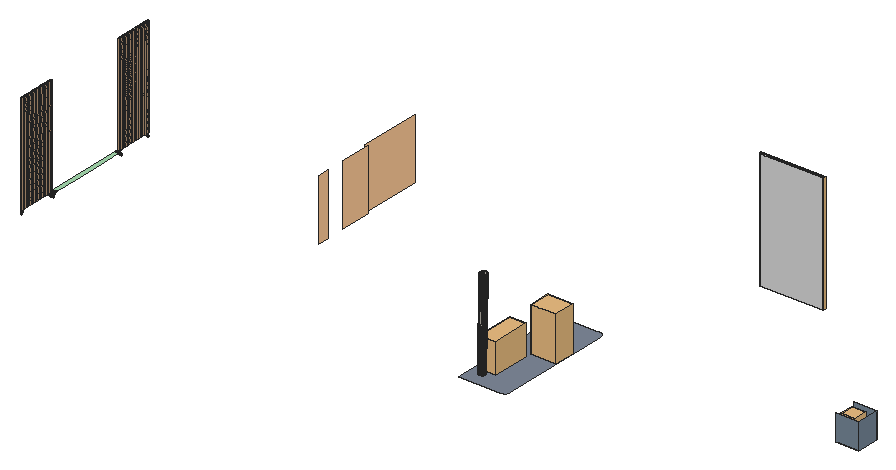
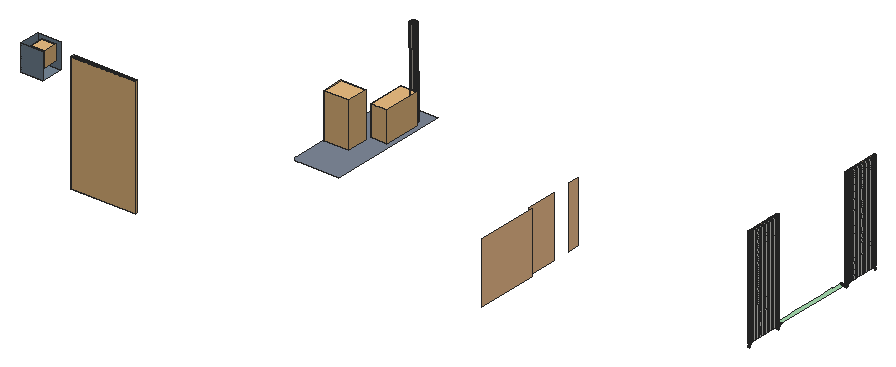
# SketchUp Ruby script. Lengths in inches.
U = 1.inch
M = Sketchup.active_model
def pt(a) = Geom::Point3d.new(a.map { |v| v * U })
def face(e, loops, mat)
  f = e.add_face(loops[0].map { |a| pt(a) })
  loops[1..].each { |l| e.add_face(l.map { |a| pt(a) }).erase! }
  f.material = f.back_material = mat if mat
  f
end
# faces: each face lists its corners as indices into pts; further lists are holes
def faces(e, pts, list, mat = nil) = list.each { |f| face(e, (f[0].is_a?(Array) ? f : [f]).map { |l| l.map { |i| pts[i] } }, mat) }
# xy, xz, yz: faces in a plane at the given z, y or x. An outline is a flat list of corners, or four numbers for a rectangle; further outlines are holes
def ring(l) = l.size == 4 ? [[l[0], l[1]], [l[2], l[1]], [l[2], l[3]], [l[0], l[3]]] : l.each_slice(2).to_a
def flat(e, list, mat, &to3) = list.each { |f| face(e, (f[0].is_a?(Array) ? f : [f]).map { |l| ring(l).map { |u, v| to3.(u, v) } }, mat) }
def xy(e, z, list, mat = nil) = flat(e, list, mat) { |x, y| [x, y, z] }
def xz(e, y, list, mat = nil) = flat(e, list, mat) { |x, z| [x, y, z] }
def yz(e, x, list, mat = nil) = flat(e, list, mat) { |y, z| [x, y, z] }
def lines(e, pts, list) = list.each { |a, b| e.add_line(pt(pts[a]), pt(pts[b])) }
# prism: a flat outline (further loops are holes) pulled along v
def prism(e, loops, v, mat = nil)
  f = face(e, loops, mat); d = Geom::Vector3d.new(v.map { |x| x * U })
  f.pushpull(f.normal.samedirection?(d) ? d.length : -d.length)
end
def box(e, o, s, mat = nil) = prism(e, [[o, [o[0] + s[0], o[1], o[2]], [o[0] + s[0], o[1] + s[1], o[2]], [o[0], o[1] + s[1], o[2]]]], [0, 0, s[2]], mat)
def at(x, y, z, deg = 0) = Geom::Transformation.translation(pt([x, y, z])) * Geom::Transformation.rotation(ORIGIN, Z_AXIS, deg.degrees)
def axes(o, x, y, z) = Geom::Transformation.new([*x, 0, *y, 0, *z, 0, *pt(o).to_a, 1])
def part(name) = M.definitions.add(name)
# library, detail: a bought-in or finely detailed component or shape, given as its bounding box
def library(name, o, s) = part(name).tap { |d| box(d.entities, o, s) }
def detail(e, o, s) = box(e.add_group.entities, o, s)
def put(e, d, t, mat = nil) = e.add_instance(d, t).tap { |i| i.material = mat if mat }
def group(e, t, mat = nil) = e.add_group.tap { |g| g.transformation = t; g.material = mat if mat }.entities
root = M.entities
M.materials.add("Leather K01 Brown 12cm").color = [167, 219, 175]
M.materials.add("Plywood B 50cm").color = [193, 159, 125]
M.materials.add("Stone E 150cm").color = [186, 180, 170]
M.materials.add("[0110_LightSlateGray]").color = [127, 136, 153]
M.materials.add("[0110_LightSlateGray]1").color = [119, 136, 153]
M.materials.add("[Color A01]1").color = [216, 216, 216]
M.materials.add("[Color C02]").color = [255, 204, 153]
c1 = library("Group\#9",[-0.5,-0.5,0],[47.92,1.3125,88])
c2 = library("Books 120 040",[-9.2,-4.08,-0.03],[18.37,8.13,11.52])
c3 = library("Vase 160 010",[-6.09,-4.45,0],[12.18,8.9,22.13])
c4 = library("Spot Light\#1",[-5.1,-5.1,-11.05],[10.2,10.2,11.05])
xy(root,57.82,[[536.14,116.57,553.2,132.48]],"[0110_LightSlateGray]1")
xy(root,62.4375,[[391.15,226.6,438.07,227.79]],"[Color A01]1")
xy(root,63.71,[[[323.37,31.6,353.74,31.6,354.39,31.64,355.03,31.75,355.65,31.9375,356.24,32.19,356.78,32.51,357.28,32.89,357.71,33.33,358.07,33.8,358.36,34.32,358.57,34.86,358.7,35.43,358.74,36,358.74,119.11,358.7,119.68,358.57,120.25,358.36,120.79,358.07,121.31,357.71,121.79,357.28,122.22,356.78,122.6,356.24,122.92,355.65,123.17,355.03,123.36,354.39,123.47,353.74,123.51,323.37,123.51],[331.76,40.57,331.08,40.64,330.44,40.87,329.89,41.24,329.47,41.71,329.21,42.27,329.12,42.87,329.2,43.46,329.46,44.02,329.875,44.5,330.41,44.87,331.05,45.11,331.72,45.1875,332.4,45.11,333.04,44.89,333.59,44.52,334.01,44.05,334.27,43.49,334.37,42.89,334.28,42.29,334.02,41.74,333.61,41.25,333.07,40.89,332.43,40.65]]],"[0110_LightSlateGray]")
xy(root,70.0625,[[8.12,18.51,9.37,19.28],[8.12,21.51,9.37,21.77],[9.37,21.51,9.43,21.51,9.43,42.51,9.37,42.51,9.37,42.15,8.12,42.15,8.12,41.68,9.37,41.68,9.37,40.91,8.12,40.91,8.12,40.43,9.37,40.43,9.37,39.66,8.12,39.66,8.12,39.1875,9.37,39.1875,9.37,38.42,8.12,38.42,8.12,37.94,9.37,37.94,9.37,37.18,8.12,37.18,8.12,36.7,9.37,36.7,9.37,35.93,8.12,35.93,8.12,35.45,9.37,35.45,9.37,34.6875,8.12,34.6875,8.12,34.21,9.37,34.21,9.37,33.44,8.12,33.44,8.12,32.97,9.37,32.97,9.37,32.2,8.12,32.2,8.12,31.72,9.37,31.72,9.37,30.95,8.12,30.95,8.12,30.48,9.37,30.48,9.37,29.71,8.12,29.71,8.12,29.23,9.37,29.23,9.37,28.47,8.12,28.47,8.12,27.99,9.37,27.99,9.37,27.22,8.12,27.22,8.12,26.74,9.37,26.74,9.37,25.98,8.12,25.98,8.12,25.5,9.37,25.5,9.37,24.73,8.12,24.73,8.12,24.25,9.37,24.25,9.37,23.49,8.12,23.49,8.12,23.01,9.37,23.01,9.37,22.24,8.12,22.24,8.12,21.77,9.37,21.77],[8.12,22.24,9.37,23.01],[8.12,23.49,9.37,24.25],
  [8.12,24.73,9.37,25.5],[8.12,25.98,9.37,26.74],[8.12,27.22,9.37,27.99],[8.12,28.47,9.37,29.23],[8.12,29.71,9.37,30.48],
  [8.12,30.95,9.37,31.72],[8.12,32.2,9.37,32.97],[8.12,33.44,9.37,34.21],[8.12,34.6875,9.37,35.45],[8.12,35.93,9.37,36.7],
  [8.12,37.18,9.37,37.94],[8.12,38.42,9.37,39.1875],[8.12,39.66,9.37,40.43],[8.12,40.91,9.37,41.68],[8.12,42.15,9.37,42.51],
  [8.12,112.01,9.37,112.23],[8.12,112.69,9.37,113.46],[8.12,113.92,9.37,114.6875],[8.12,115.15,9.37,115.91],[8.12,116.375,9.37,117.14],
  [8.12,117.6,9.37,118.37],[8.12,118.83,9.37,119.6],[8.12,120.06,9.37,120.82],[8.12,121.28,9.37,122.05],[8.12,122.51,9.37,123.28],
  [8.12,123.74,9.37,124.5],[8.12,124.97,9.37,125.73],[8.12,126.19,9.37,126.96],[8.12,127.42,9.37,128.1875],[8.12,128.65,9.37,129.41],
  [8.12,129.875,9.37,130.64],[8.12,131.1,9.37,131.87],[8.12,132.33,9.37,133.01]])
xy(root,70.0625,[[8.12,48.51,11.43,48.51,11.43,54.26,10.74,54.26,10.74,55.26,11.43,55.26,11.43,62.26,10.74,62.26,10.74,63.26,11.43,63.26,11.43,91.64,10.74,91.64,10.74,92.64,11.43,92.64,11.43,99.64,10.74,99.64,10.74,100.64,11.43,100.64,11.43,106.01,8.12,106.01],[9.37,112.01,9.43,112.01,9.43,133.01,9.37,133.01,9.37,132.33,8.12,132.33,8.12,131.87,9.37,131.87,9.37,131.1,8.12,131.1,8.12,130.64,9.37,130.64,9.37,129.875,8.12,129.875,8.12,129.41,9.37,129.41,9.37,128.65,8.12,128.65,8.12,128.1875,9.37,128.1875,9.37,127.42,8.12,127.42,8.12,126.96,9.37,126.96,9.37,126.19,8.12,126.19,8.12,125.73,9.37,125.73,9.37,124.97,8.12,124.97,8.12,124.5,9.37,124.5,9.37,123.74,8.12,123.74,8.12,123.28,9.37,123.28,9.37,122.51,8.12,122.51,8.12,122.05,9.37,122.05,9.37,121.28,8.12,121.28,8.12,120.82,9.37,120.82,9.37,120.06,8.12,120.06,8.12,119.6,9.37,119.6,9.37,118.83,8.12,118.83,8.12,118.37,9.37,118.37,9.37,117.6,8.12,117.6,8.12,117.14,9.37,117.14,9.37,116.375,8.12,116.375,8.12,115.91,9.37,115.91,9.37,115.15,8.12,115.15,8.12,114.6875,9.37,114.6875,9.37,113.92,8.12,113.92,8.12,113.46,9.37,113.46,9.37,112.69,8.12,112.69,8.12,112.23,9.37,112.23]],"Leather K01 Brown 12cm")
xy(root,144.0625,[[8.12,19.76,9.37,20.52],[8.12,43.4,9.37,44.16],[8.12,44.64,9.37,45.41],[8.12,45.89,9.37,46.65],[8.12,109.01,9.37,109.78],
  [8.12,110.24,9.37,111],[8.12,133.56,9.37,134.32],[8.12,134.78,9.37,135.55],[8.12,136.01,9.37,136.78]],"Plywood B 50cm")
xy(root,150.4375,[[391.15,226.6,438.07,227.79]],"[Color A01]1")
xz(root,18.51,[[8.12,70.0625,9.37,144.0625]],"Plywood B 50cm")
xz(root,19.28,[[8.12,70.0625,9.37,144.0625]],"Plywood B 50cm")
xz(root,19.76,[[8.12,70.0625,9.37,144.0625]],"Plywood B 50cm")
xz(root,20.52,[[8.12,70.0625,9.37,144.0625]],"Plywood B 50cm")
xz(root,21,[[8.12,70.0625,9.37,144.0625]],"Plywood B 50cm")
xz(root,21.77,[[8.12,70.0625,9.37,144.0625]],"Plywood B 50cm")
xz(root,22.24,[[8.12,70.0625,9.37,144.0625]],"Plywood B 50cm")
xz(root,23.01,[[8.12,70.0625,9.37,144.0625]],"Plywood B 50cm")
xz(root,23.49,[[8.12,70.0625,9.37,144.0625]],"Plywood B 50cm")
xz(root,24.25,[[8.12,70.0625,9.37,144.0625]],"Plywood B 50cm")
xz(root,24.73,[[8.12,70.0625,9.37,144.0625]],"Plywood B 50cm")
xz(root,25.5,[[8.12,70.0625,9.37,144.0625]])
xz(root,25.98,[[8.12,70.0625,9.37,144.0625]],"Plywood B 50cm")
xz(root,26.74,[[8.12,70.0625,9.37,144.0625]],"Plywood B 50cm")
xz(root,27.22,[[8.12,70.0625,9.37,144.0625]],"Plywood B 50cm")
xz(root,27.99,[[8.12,70.0625,9.37,144.0625]],"Plywood B 50cm")
xz(root,28.47,[[8.12,70.0625,9.37,144.0625]],"Plywood B 50cm")
xz(root,29.23,[[8.12,70.0625,9.37,144.0625]],"Plywood B 50cm")
xz(root,29.71,[[8.12,70.0625,9.37,144.0625]],"Plywood B 50cm")
xz(root,30.48,[[8.12,70.0625,9.37,144.0625]],"Plywood B 50cm")
xz(root,30.95,[[8.12,70.0625,9.37,144.0625]],"Plywood B 50cm")
xz(root,31.72,[[8.12,70.0625,9.37,144.0625]],"Plywood B 50cm")
xz(root,32.2,[[8.12,70.0625,9.37,144.0625]],"Plywood B 50cm")
xz(root,32.97,[[8.12,70.0625,9.37,144.0625]],"Plywood B 50cm")
xz(root,33.44,[[8.12,70.0625,9.37,144.0625]],"Plywood B 50cm")
xz(root,34.21,[[8.12,70.0625,9.37,144.0625]],"Plywood B 50cm")
xz(root,34.6875,[[8.12,70.0625,9.37,144.0625]],"Plywood B 50cm")
xz(root,35.45,[[8.12,70.0625,9.37,144.0625]],"Plywood B 50cm")
xz(root,35.93,[[8.12,70.0625,9.37,144.0625]],"Plywood B 50cm")
xz(root,36.7,[[8.12,70.0625,9.37,144.0625]],"Plywood B 50cm")
xz(root,37.18,[[8.12,70.0625,9.37,144.0625]],"Plywood B 50cm")
xz(root,37.94,[[8.12,70.0625,9.37,144.0625]],"Plywood B 50cm")
xz(root,38.42,[[8.12,70.0625,9.37,144.0625]],"Plywood B 50cm")
xz(root,39.1875,[[8.12,70.0625,9.37,144.0625]],"Plywood B 50cm")
xz(root,39.66,[[8.12,70.0625,9.37,144.0625]],"Plywood B 50cm")
xz(root,40.43,[[8.12,70.0625,9.37,144.0625]],"Plywood B 50cm")
xz(root,40.91,[[8.12,70.0625,9.37,144.0625]],"Plywood B 50cm")
xz(root,41.68,[[8.12,70.0625,9.37,144.0625]],"Plywood B 50cm")
xz(root,42.15,[[8.12,70.0625,9.37,144.0625]],"Plywood B 50cm")
xz(root,42.92,[[8.12,70.0625,9.37,144.0625]],"Plywood B 50cm")
xz(root,43.4,[[8.12,70.0625,9.37,144.0625]],"Plywood B 50cm")
xz(root,44.16,[[8.12,70.0625,9.37,144.0625]],"Plywood B 50cm")
xz(root,44.64,[[8.12,70.0625,9.37,144.0625]],"Plywood B 50cm")
xz(root,45.41,[[8.12,70.0625,9.37,144.0625]],"Plywood B 50cm")
xz(root,45.89,[[8.12,70.0625,9.37,144.0625]],"Plywood B 50cm")
xz(root,46.65,[[8.12,70.0625,9.37,144.0625]],"Plywood B 50cm")
xz(root,109.01,[[8.12,70.0625,9.37,144.0625]],"Plywood B 50cm")
xz(root,109.78,[[8.12,70.0625,9.37,144.0625]],"Plywood B 50cm")
xz(root,110.24,[[8.12,70.0625,9.37,144.0625]],"Plywood B 50cm")
xz(root,111,[[8.12,70.0625,9.37,144.0625]],"Plywood B 50cm")
xz(root,111.47,[[8.12,70.0625,9.37,144.0625]],"Plywood B 50cm")
xz(root,112.23,[[8.12,70.0625,9.37,144.0625]],"Plywood B 50cm")
xz(root,112.69,[[8.12,70.0625,9.37,144.0625]],"Plywood B 50cm")
xz(root,113.46,[[8.12,70.0625,9.37,144.0625]],"Plywood B 50cm")
xz(root,113.92,[[8.12,70.0625,9.37,144.0625]],"Plywood B 50cm")
xz(root,114.6875,[[8.12,70.0625,9.37,144.0625]],"Plywood B 50cm")
xz(root,115.15,[[8.12,70.0625,9.37,144.0625]],"Plywood B 50cm")
xz(root,115.91,[[8.12,70.0625,9.37,144.0625]],"Plywood B 50cm")
xz(root,116.375,[[8.12,70.0625,9.37,144.0625]],"Plywood B 50cm")
xz(root,116.57,[[536.14,57.82,553.2,76.9375]],"[0110_LightSlateGray]1")
xz(root,117.14,[[8.12,70.0625,9.37,144.0625]],"Plywood B 50cm")
xz(root,117.6,[[8.12,70.0625,9.37,144.0625]],"Plywood B 50cm")
xz(root,118.37,[[8.12,70.0625,9.37,144.0625]],"Plywood B 50cm")
xz(root,118.83,[[8.12,70.0625,9.37,144.0625]],"Plywood B 50cm")
xz(root,119.6,[[8.12,70.0625,9.37,144.0625]],"Plywood B 50cm")
xz(root,120.06,[[8.12,70.0625,9.37,144.0625]],"Plywood B 50cm")
xz(root,120.82,[[8.12,70.0625,9.37,144.0625]],"Plywood B 50cm")
xz(root,121.28,[[8.12,70.0625,9.37,144.0625]],"Plywood B 50cm")
xz(root,122.05,[[8.12,70.0625,9.37,144.0625]],"Plywood B 50cm")
xz(root,122.51,[[8.12,70.0625,9.37,144.0625]],"Plywood B 50cm")
xz(root,123.28,[[8.12,70.0625,9.37,144.0625]],"Plywood B 50cm")
xz(root,123.74,[[8.12,70.0625,9.37,144.0625]],"Plywood B 50cm")
xz(root,124.5,[[8.12,70.0625,9.37,144.0625]],"Plywood B 50cm")
xz(root,124.97,[[8.12,70.0625,9.37,144.0625]],"Plywood B 50cm")
xz(root,125.73,[[8.12,70.0625,9.37,144.0625]],"Plywood B 50cm")
xz(root,126.19,[[8.12,70.0625,9.37,144.0625]],"Plywood B 50cm")
xz(root,126.96,[[8.12,70.0625,9.37,144.0625]],"Plywood B 50cm")
xz(root,127.42,[[8.12,70.0625,9.37,144.0625]],"Plywood B 50cm")
xz(root,128.1875,[[8.12,70.0625,9.37,144.0625]],"Plywood B 50cm")
xz(root,128.65,[[8.12,70.0625,9.37,144.0625]],"Plywood B 50cm")
xz(root,129.41,[[8.12,70.0625,9.37,144.0625]])
xz(root,129.875,[[8.12,70.0625,9.37,144.0625]],"Plywood B 50cm")
xz(root,130.64,[[8.12,70.0625,9.37,144.0625]],"Plywood B 50cm")
xz(root,131.1,[[8.12,70.0625,9.37,144.0625]],"Plywood B 50cm")
xz(root,131.87,[[8.12,70.0625,9.37,144.0625]],"Plywood B 50cm")
xz(root,132.33,[[8.12,70.0625,9.37,144.0625]],"Plywood B 50cm")
xz(root,132.48,[[536.14,57.82,553.2,76.9375]],"[0110_LightSlateGray]1")
xz(root,133.1,[[8.12,70.0625,9.37,144.0625]],"Plywood B 50cm")
xz(root,133.56,[[8.12,70.0625,9.37,144.0625]],"Plywood B 50cm")
xz(root,134.32,[[8.12,70.0625,9.37,144.0625]],"Plywood B 50cm")
xz(root,134.78,[[8.12,70.0625,9.37,144.0625]],"Plywood B 50cm")
xz(root,135.55,[[8.12,70.0625,9.37,144.0625]],"Plywood B 50cm")
xz(root,136.01,[[8.12,70.0625,9.37,144.0625]],"Plywood B 50cm")
xz(root,136.78,[[8.12,70.0625,9.37,144.0625]],"Plywood B 50cm")
xz(root,226.6,[[391.15,62.4375,438.07,150.4375]],"[Color A01]1")
xz(root,228.1,[[391.15,62.4375,438.07,150.4375]])
yz(root,8.12,[[22.24,70.0625,23.01,144.0625],[23.49,70.0625,24.25,144.0625],[24.73,70.0625,25.5,144.0625],[25.98,70.0625,26.74,144.0625],[27.22,70.0625,27.99,144.0625],
  [28.47,70.0625,29.23,144.0625],[29.71,70.0625,30.48,144.0625],[30.95,70.0625,31.72,144.0625],[32.2,70.0625,32.97,144.0625],[33.44,70.0625,34.21,144.0625],
  [34.6875,70.0625,35.45,144.0625],[35.93,70.0625,36.7,144.0625],[37.18,70.0625,37.94,144.0625],[38.42,70.0625,39.1875,144.0625],[39.66,70.0625,40.43,144.0625],
  [40.91,70.0625,41.68,144.0625],[112.69,70.0625,113.46,144.0625],[113.92,70.0625,114.6875,144.0625],[115.15,70.0625,115.91,144.0625],[116.375,70.0625,117.14,144.0625],
  [117.6,70.0625,118.37,144.0625],[118.83,70.0625,119.6,144.0625],[120.06,70.0625,120.82,144.0625],[121.28,70.0625,122.05,144.0625],[122.51,70.0625,123.28,144.0625],
  [123.74,70.0625,124.5,144.0625],[124.97,70.0625,125.73,144.0625],[126.19,70.0625,126.96,144.0625],[127.42,70.0625,128.1875,144.0625],[128.65,70.0625,129.41,144.0625],
  [129.875,70.0625,130.64,144.0625],[131.1,70.0625,131.87,144.0625]])
yz(root,9.37,[[18.51,70.0625,19.28,144.0625],[19.76,70.0625,20.52,144.0625],[21,70.0625,21.77,144.0625],[22.24,70.0625,23.01,144.0625],[23.49,70.0625,24.25,144.0625],
  [24.73,70.0625,25.5,144.0625],[25.98,70.0625,26.74,144.0625],[27.22,70.0625,27.99,144.0625],[28.47,70.0625,29.23,144.0625],[29.71,70.0625,30.48,144.0625],
  [30.95,70.0625,31.72,144.0625],[32.2,70.0625,32.97,144.0625],[33.44,70.0625,34.21,144.0625],[34.6875,70.0625,35.45,144.0625],[35.93,70.0625,36.7,144.0625],
  [37.18,70.0625,37.94,144.0625],[38.42,70.0625,39.1875,144.0625],[39.66,70.0625,40.43,144.0625],[40.91,70.0625,41.68,144.0625],[42.15,70.0625,42.92,144.0625],
  [43.4,70.0625,44.16,144.0625],[44.64,70.0625,45.41,144.0625],[45.89,70.0625,46.65,144.0625],[109.01,70.0625,109.78,144.0625],[110.24,70.0625,111,144.0625],
  [111.47,70.0625,112.23,144.0625],[112.69,70.0625,113.46,144.0625],[113.92,70.0625,114.6875,144.0625],[115.15,70.0625,115.91,144.0625],[116.375,70.0625,117.14,144.0625],
  [117.6,70.0625,118.37,144.0625],[118.83,70.0625,119.6,144.0625],[120.06,70.0625,120.82,144.0625],[121.28,70.0625,122.05,144.0625],[122.51,70.0625,123.28,144.0625],
  [123.74,70.0625,124.5,144.0625],[124.97,70.0625,125.73,144.0625],[126.19,70.0625,126.96,144.0625],[127.42,70.0625,128.1875,144.0625],[128.65,70.0625,129.41,144.0625],
  [129.875,70.0625,130.64,144.0625],[131.1,70.0625,131.87,144.0625],[132.33,70.0625,133.1,144.0625],[133.56,70.0625,134.32,144.0625],[134.78,70.0625,135.55,144.0625],
  [136.01,70.0625,136.78,144.0625]],"Plywood B 50cm")
yz(root,161.57,[[147.01,65.06,192.875,110.51]],"[Color C02]")
yz(root,163.32,[[101.5625,65.06,109.82,110.51],[124.45,65.06,147.01,110.51]],"[Color C02]")
yz(root,391.15,[[226.6,62.4375,227.79,150.4375]],"[Color A01]1")
yz(root,438.07,[[226.6,62.4375,227.79,150.4375]],"[Color A01]1")
yz(root,553.2,[[116.57,57.82,132.48,76.9375]],"[0110_LightSlateGray]1")
p = [[331.08,40.64,63.71],[331.08,41.875,129.78],[330.44,40.87,63.71],[331.76,40.57,63.71],[331.76,41.79,129.78],[332.43,40.65,63.71],
  [332.43,41.88,129.78],[333.07,40.89,63.71],[333.07,42.15,129.78],[330.44,42.14,129.78],[329.89,41.24,63.71],[333.61,41.25,63.71],
  [333.61,42.57,129.78],[329.89,42.55,129.78],[329.47,43.09,129.78],[329.47,41.71,63.71],[334.02,41.74,63.71],[329.21,43.72,129.78],
  [329.21,42.27,63.71],[334.02,43.12,129.78],[334.28,42.29,63.71],[329.12,44.4,129.78],[329.12,42.87,63.71],[334.28,43.75,129.78],
  [334.37,42.89,63.71],[329.2,45.08,129.78],[329.2,43.46,63.71],[334.37,44.43,129.78],[334.27,43.49,63.71],[329.46,45.72,129.78],
  [329.46,44.02,63.71],[334.01,44.05,63.71],[334.27,45.11,129.78],[329.875,46.26,129.78],[329.875,44.5,63.71],[333.59,44.52,63.71],
  [334.01,45.74,129.78],[330.41,44.87,63.71],[333.04,44.89,63.71],[333.04,46.7,129.78],[333.59,46.28,129.78],[330.41,46.68,129.78],
  [331.05,45.11,63.71],[332.4,45.11,63.71],[332.4,46.96,129.78],[331.05,46.95,129.78],[331.72,45.1875,63.71],[331.72,47.04,129.78],
  [8.12,18.54,67.45],[8.12,18.51,67.0625],[9.43,18.51,67.0625],[9.43,18.54,67.45],[8.12,45.51,67.0625],[8.12,45.49,67.45],
  [9.43,45.49,67.45],[9.43,45.51,67.0625],[8.12,45.54,67.45],[11.43,45.51,67.0625],[11.43,45.54,67.45],[8.12,109.01,67.0625],
  [8.12,108.99,67.45],[11.43,108.99,67.45],[11.43,109.01,67.0625],[9.43,109.01,67.0625],[8.12,109.04,67.45],[9.43,109.04,67.45],
  [8.12,136.01,67.0625],[8.12,135.99,67.45],[9.43,135.99,67.45],[9.43,136.01,67.0625],[8.12,18.61,67.84],[9.43,18.61,67.84],
  [8.12,45.41,67.84],[9.43,45.41,67.84],[8.12,45.61,67.84],[11.43,45.61,67.84],[8.12,108.91,67.84],[11.43,108.91,67.84],
  [8.12,109.11,67.84],[9.43,109.11,67.84],[8.12,135.91,67.84],[9.43,135.91,67.84],[8.12,18.74,68.21],[9.43,18.74,68.21],
  [8.12,45.28,68.21],[9.43,45.28,68.21],[8.12,45.74,68.21],[11.43,45.74,68.21],[8.12,108.78,68.21],[11.43,108.78,68.21],
  [8.12,109.24,68.21],[9.43,109.24,68.21],[8.12,135.78,68.21],[9.43,135.78,68.21],[8.12,18.91,68.5625],[9.43,18.91,68.5625],
  [8.12,45.11,68.5625],[9.43,45.11,68.5625],[8.12,45.91,68.5625],[11.43,45.91,68.5625],[8.12,108.61,68.5625],[11.43,108.61,68.5625],
  [8.12,109.41,68.5625],[9.43,109.41,68.5625],[8.12,135.61,68.5625],[9.43,135.61,68.5625],[8.12,19.13,68.89],[9.43,19.13,68.89],
  [8.12,44.89,68.89],[9.43,44.89,68.89],[8.12,46.13,68.89],[11.43,46.13,68.89],[8.12,108.39,68.89],[11.43,108.39,68.89],
  [8.12,109.63,68.89],[9.43,109.63,68.89],[8.12,135.39,68.89],[9.43,135.39,68.89],[8.12,19.39,69.18],[9.43,19.39,69.18],
  [8.12,44.63,69.18],[9.43,44.63,69.18],[8.12,46.39,69.18],[11.43,46.39,69.18],[8.12,108.13,69.18],[11.43,108.13,69.18],
  [8.12,109.89,69.18],[9.43,109.89,69.18],[8.12,135.13,69.18],[9.43,135.13,69.18],[8.12,19.68,69.44],[9.43,19.68,69.44],
  [8.12,44.34,69.44],[9.43,44.34,69.44],[8.12,46.68,69.44],[11.43,46.68,69.44],[8.12,107.84,69.44],[11.43,107.84,69.44],
  [8.12,110.18,69.44],[9.43,110.18,69.44],[8.12,134.84,69.44],[9.43,134.84,69.44],[8.12,20.01,69.66],[9.43,20.01,69.66],
  [8.12,44.01,69.66],[9.43,44.01,69.66],[8.12,47.01,69.66],[11.43,47.01,69.66],[8.12,107.51,69.66],[11.43,107.51,69.66],
  [8.12,110.51,69.66],[9.43,110.51,69.66],[8.12,134.51,69.66],[9.43,134.51,69.66],[8.12,20.36,69.83],[9.43,20.36,69.83],
  [8.12,43.66,69.83],[9.43,43.66,69.83],[8.12,47.36,69.83],[11.43,47.36,69.83],[8.12,107.16,69.83],[11.43,107.16,69.83],
  [8.12,110.86,69.83],[9.43,110.86,69.83],[8.12,134.16,69.83],[9.43,134.16,69.83],[8.12,20.73,69.96],[9.43,20.73,69.96],
  [8.12,43.29,69.96],[9.43,43.29,69.96],[8.12,47.73,69.96],[11.43,47.73,69.96],[8.12,106.79,69.96],[11.43,106.79,69.96],
  [8.12,111.23,69.96],[9.43,111.23,69.96],[8.12,133.79,69.96],[9.43,133.79,69.96],[8.12,21.12,70.04],[9.43,21.12,70.04],
  [8.12,21.51,70.0625],[9.43,21.51,70.0625],[9.37,21.51,70.0625],[8.12,42.9,70.04],[8.12,42.51,70.0625],[9.37,42.51,70.0625],
  [9.43,42.51,70.0625],[9.43,42.9,70.04],[8.12,48.12,70.04],[11.43,48.12,70.04],[8.12,48.51,70.0625],[11.43,48.51,70.0625],
  [8.12,106.4,70.04],[8.12,106.01,70.0625],[11.43,106.01,70.0625],[11.43,106.4,70.04],[8.12,111.62,70.04],[9.43,111.62,70.04],
  [8.12,112.01,70.0625],[9.43,112.01,70.0625],[9.37,112.01,70.0625],[8.12,133.4,70.04],[8.12,133.01,70.0625],[9.37,133.01,70.0625],
  [9.43,133.01,70.0625],[9.43,133.4,70.04]]
faces(root,p,[[0,1,2],[3,4,0],[1,0,4],[5,6,3],[4,3,6],[7,8,5],[6,5,8],[2,9,10],
  [9,2,1],[11,12,7],[8,7,12],[13,14,10],[15,10,14],[13,10,9],[11,16,12],[14,17,15],
  [18,15,17],[19,12,16],[16,20,19],[17,21,18],[22,18,21],[23,19,20],[20,24,23],[21,25,22],
  [26,22,25],[27,23,24],[24,28,27],[25,29,26],[30,26,29],[28,31,32],[32,27,28],[29,33,30],
  [34,30,33],[31,35,36],[36,32,31],[34,33,37],[38,39,35],[40,35,39],[40,36,35],[41,37,33],
  [37,41,42],[43,44,38],[39,38,44],[45,42,41],[42,45,46],[46,47,43],[44,43,47],[47,46,45]],"Stone E 150cm")
faces(root,p,[[48,49,50,51],[56,52,55,57,58],[59,60,61,62,63],[64,59,63,65],[66,67,68,69],[70,48,51,71],[74,56,58,75],[60,76,77,61],
  [78,64,65,79],[67,80,81,68],[82,70,71,83],[86,74,75,87],[76,88,89,77],[90,78,79,91],[80,92,93,81],[94,82,83,95],
  [98,86,87,99],[88,100,101,89],[102,90,91,103],[92,104,105,93],[106,94,95,107],[110,98,99,111],[100,112,113,101],[114,102,103,115],
  [104,116,117,105],[118,106,107,119],[122,110,111,123],[112,124,125,113],[126,114,115,127],[116,128,129,117],[130,118,119,131],[134,122,123,135],
  [124,136,137,125],[138,126,127,139],[128,140,141,129],[142,130,131,143],[146,134,135,147],[136,148,149,137],[150,138,139,151],[140,152,153,141],
  [154,142,143,155],[158,146,147,159],[148,160,161,149],[162,150,151,163],[152,164,165,153],[166,154,155,167],[170,158,159,171],[160,172,173,161],
  [174,162,163,175],[164,176,177,165],[178,166,167,179],[180,178,179,181,182],[188,170,171,189],[190,188,189,191],[192,193,194,195],[172,192,195,173],
  [196,174,175,197],[198,196,197,199,200],[201,202,203,204,205],[176,201,205,177]],"Leather K01 Brown 12cm")
faces(root,p,[[52,53,54,55],[53,72,73,54],[72,84,85,73],[84,96,97,85],[96,108,109,97],[108,120,121,109],[120,132,133,121],[132,144,145,133],
  [144,156,157,145],[156,168,169,157],[183,184,185,186,187],[168,183,187,169]])
put(root,c1,at(391.15,227.79,62.4375))
put(root,c2,axes([333.24,60.43,63.68],[0,1.5,0],[-1.5,0,0],[0,0,1.95]))
put(root,c3,axes([348.9,86.24,63.71],[1.5,0,0],[0,1.77,0],[0,0,1.5]))
put(root,c4,at(542.65,124.62,75.86))
